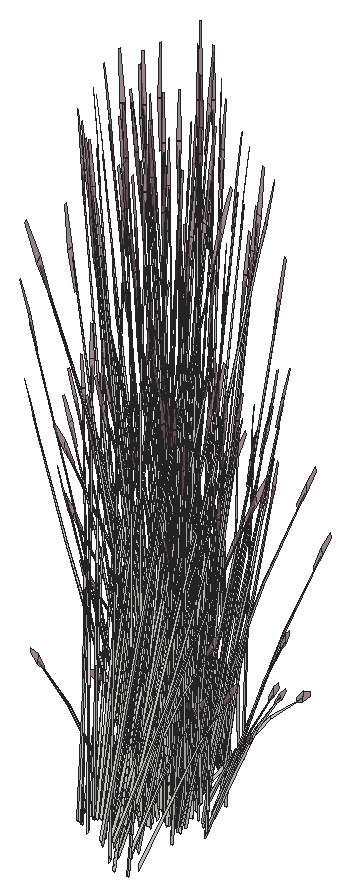
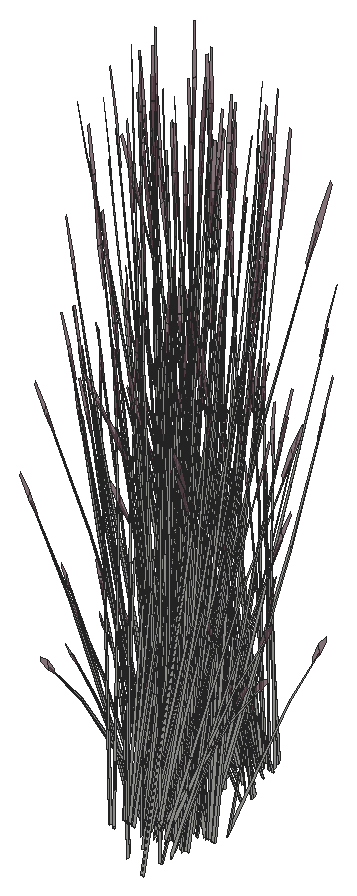
# SketchUp Ruby script. Lengths in inches.
U = 1.inch
M = Sketchup.active_model
def pt(a) = Geom::Point3d.new(a.map { |v| v * U })
def face(e, loops, mat)
  f = e.add_face(loops[0].map { |a| pt(a) })
  loops[1..].each { |l| e.add_face(l.map { |a| pt(a) }).erase! }
  f.material = f.back_material = mat if mat
  f
end
# faces: each face lists its corners as indices into pts; further lists are holes
def faces(e, pts, list, mat = nil) = list.each { |f| face(e, (f[0].is_a?(Array) ? f : [f]).map { |l| l.map { |i| pts[i] } }, mat) }
# xy, xz, yz: faces in a plane at the given z, y or x. An outline is a flat list of corners, or four numbers for a rectangle; further outlines are holes
def ring(l) = l.size == 4 ? [[l[0], l[1]], [l[2], l[1]], [l[2], l[3]], [l[0], l[3]]] : l.each_slice(2).to_a
def flat(e, list, mat, &to3) = list.each { |f| face(e, (f[0].is_a?(Array) ? f : [f]).map { |l| ring(l).map { |u, v| to3.(u, v) } }, mat) }
def xy(e, z, list, mat = nil) = flat(e, list, mat) { |x, y| [x, y, z] }
def xz(e, y, list, mat = nil) = flat(e, list, mat) { |x, z| [x, y, z] }
def yz(e, x, list, mat = nil) = flat(e, list, mat) { |y, z| [x, y, z] }
def lines(e, pts, list) = list.each { |a, b| e.add_line(pt(pts[a]), pt(pts[b])) }
# prism: a flat outline (further loops are holes) pulled along v
def prism(e, loops, v, mat = nil)
  f = face(e, loops, mat); d = Geom::Vector3d.new(v.map { |x| x * U })
  f.pushpull(f.normal.samedirection?(d) ? d.length : -d.length)
end
def box(e, o, s, mat = nil) = prism(e, [[o, [o[0] + s[0], o[1], o[2]], [o[0] + s[0], o[1] + s[1], o[2]], [o[0], o[1] + s[1], o[2]]]], [0, 0, s[2]], mat)
def at(x, y, z, deg = 0) = Geom::Transformation.translation(pt([x, y, z])) * Geom::Transformation.rotation(ORIGIN, Z_AXIS, deg.degrees)
def axes(o, x, y, z) = Geom::Transformation.new([*x, 0, *y, 0, *z, 0, *pt(o).to_a, 1])
def part(name) = M.definitions.add(name)
# library, detail: a bought-in or finely detailed component or shape, given as its bounding box
def library(name, o, s) = part(name).tap { |d| box(d.entities, o, s) }
def detail(e, o, s) = box(e.add_group.entities, o, s)
def put(e, d, t, mat = nil) = e.add_instance(d, t).tap { |i| i.material = mat if mat }
def group(e, t, mat = nil) = e.add_group.tap { |g| g.transformation = t; g.material = mat if mat }.entities
root = M.entities
M.materials.add("LightPink_Translucent").color = [144, 107, 117]
M.materials["LightPink_Translucent"].alpha = 0.75
c1 = part("blade")
p = [[2.15,0.21,22],[0,0.17,0],[0.09,0.45,0],[2.18,0.31,22],[2.29,0.31,22],[0.38,0.45,0],
  [2.48,0.24,33],[2.49,0.24,33],[2.48,0.22,33]]
faces(c1.entities,p,[[0,1,2,3],[4,5,2,3],[6,3,4,7],[8,0,3,6]])
c2 = part("seeds")
p = [[0.3,-0.1,1.38],[-0.01,-0.03,1.59],[-0.01,-0.03,0.03],[0.14,-0.07,-0.07],[0.29,-0.03,3],[0.15,0.01,3.11]]
faces(c2.entities,p,[[0,1,2,3],[1,0,4,5]],"LightPink_Translucent")
c3 = part("blade with seeds")
put(c3.entities,c1,at(0,0,0))
put(c3.entities,c2,axes([2.4,0.25,30.99],[1.5799,-0.05474,1.17369],[-0.12525,1.92788,0.29478],[-0.07173,-0.02425,1.56792]))
put(root,c3,axes([413.54,297.29,-10.12],[0,0.54355,-0.46235],[-0.57217,0,0],[0,0.1238,1.46668]))
put(root,c3,axes([412.11,297.35,-8.39],[-0.18996,-0.09365,1.59586],[0.39312,-0.39287,0.12904],[0.24502,0.17723,0.68222]))
put(root,c3,axes([412.15,296.12,-7.83],[-0.44191,-0.28242,1.28769],[0.46662,-0.43971,0.5556],[0.14258,0.26499,1.24467]))
put(root,c3,axes([408.96,297.3125,-7.3125],[0.47307,0.29971,-0.11324],[-0.27254,0.43404,-0.62851],[-0.13365,0.15087,0.95501]))
put(root,c3,axes([412.8125,298.42,-9.42],[-0.28795,-0.15629,1.06958],[0.37181,-0.1588,0.78586],[0.10029,0.13452,0.23558]))
put(root,c3,axes([411.8,298.87,-7.3125],[0.30474,-0.46525,-0.11324],[0.44133,0.26804,-0.62851],[0.15341,0.13145,0.95501]))
put(root,c3,axes([409.82,303.12,-7.6],[0.23243,-0.34529,0.05988],[0.331,0.20103,0.47138],[-0.10701,-0.1107,0.71878]))
put(root,c3,axes([408.92,303.07,-10.61],[-0.04954,0.0716,1.6421],[-0.50062,0.15438,-0.25086],[-0.12094,-0.14044,0.2797]))
put(root,c3,axes([409.75,305.04,-10.05],[-0.21003,-0.55738,-0.65031],[0.60499,-0.20074,-0.17068],[-0.02321,-0.18874,1.43544]))
put(root,c3,axes([409.2,297.67,-7.64],[0.13138,0.49631,-0.47583],[-0.49754,0.08682,-0.36857],[-0.14258,0.13331,0.91046]))
put(root,c3,axes([412.56,303.33,-10.61],[-0.07655,-0.04282,1.6421],[-0.19662,-0.47839,-0.25086],[0.13264,-0.12982,0.2797]))
put(root,c3,axes([409.79,298.24,-7.3],[0.34603,-0.28618,0.32977],[0.32756,0.32677,-0.42575],[-0.04984,0.16603,0.81462]))
put(root,c3,axes([412.38,298.82,-9.79],[0.31974,0.54466,0],[-0.53494,0.30375,-0.48057],[-0.12184,0.06918,1.52448]))
put(root,c3,axes([410.98,303.44,-7.3],[-0.15418,0.41799,0.32977],[-0.44981,-0.12192,-0.42575],[-0.04124,-0.16829,0.81462]))
put(root,c3,axes([411.4,299.25,-7.62],[0.00151,-0.06581,1.65179],[0.43826,-0.29033,-0.15608],[0.15223,0.10363,0.29231]))
put(root,c3,axes([412.89,299,-10.61],[0.03726,-0.07847,1.6421],[0.46909,-0.23111,-0.25086],[0.14221,0.11962,0.2797]))
put(root,c3,axes([412.11,296.66,-9.35],[-0.01397,-0.51177,1.31553],[0.63227,0.13266,0.557],[-0.14954,0.28003,1.24175]))
put(root,c3,axes([412.27,297.22,-10.05],[0.18752,0.49766,-0.6445],[-0.54017,0.17923,-0.16915],[0.02073,0.16852,1.42262]))
put(root,c3,axes([409.48,298.5,-7.6],[-0.42027,-0.02533,0.05988],[0.01152,-0.38243,0.47138],[-0.04398,0.14649,0.71878]))
put(root,c3,axes([409.58,303.52,-7.64],[-0.50465,0.12921,-0.47583],[-0.08828,-0.48932,-0.36857],[-0.13555,-0.14022,0.91046]))
put(root,c3,axes([412.125,303.62,-7.59],[0.36417,0.37086,0.447],[-0.38674,0.31985,0.36857],[0.06718,-0.174,0.92496]))
put(root,c3,axes([409.61,298.53,-7.59],[-0.36417,-0.37086,0.447],[0.38674,-0.31985,0.36857],[-0.06718,0.174,0.92496]))
put(root,c3,axes([412.16,298.64,-7.64],[0.50465,-0.12921,-0.47583],[0.08828,0.48932,-0.36857],[0.13555,0.14022,0.91046]))
put(root,c3,axes([409.93,303.08,-6.94],[-0.34131,0.52108,-0.12682],[-0.49429,-0.3002,-0.70393],[-0.17182,-0.14722,1.06961]))
put(root,c3,axes([412.26,303.65,-7.6],[0.42027,0.02533,0.05988],[-0.01152,0.38243,0.47138],[0.04398,-0.14649,0.71878]))
put(root,c3,axes([410.76,298.71,-7.3],[0.15418,-0.41799,0.32977],[0.44981,0.12192,-0.42575],[0.04124,0.16829,0.81462]))
put(root,c3,axes([411.95,303.91,-7.3],[-0.34603,0.28618,0.32977],[-0.32756,-0.32677,-0.42575],[0.04984,-0.16603,0.81462]))
put(root,c3,axes([412.56,304.68,-7.36],[0.26714,-0.42887,-0.66157],[0.46811,0.30479,0.07984],[0.1595,-0.15539,0.93586]))
put(root,c3,axes([409.67,303.43,-9.79],[-0.31974,-0.54466,0],[0.53494,-0.30375,-0.48057],[0.12184,-0.06918,1.52448]))
put(root,c3,axes([412.54,304.48,-7.64],[-0.13138,-0.49631,-0.47583],[0.49754,-0.08682,-0.36857],[0.14258,-0.13331,0.91046]))
put(root,c3,axes([412.86,299.13,-9.52],[-0.32795,-0.01705,0.97832],[0.21658,-0.36206,0.54015],[0.12956,0.12863,0.76741]))
put(root,c3,axes([410.37,302.78,-10.02],[-0.35341,0.31182,-0.03625],[-0.32382,-0.34152,-0.16435],[-0.0228,-0.09677,0.54209]))
put(root,c3,axes([411.91,299.04,-7.6],[-0.23243,0.34529,0.05988],[-0.331,-0.20103,0.47138],[0.10701,0.1107,0.71878]))
put(root,c3,axes([411.37,300.2,-6.74],[0.35341,-0.31182,-0.06041],[0.32382,0.34152,-0.27392],[0.0228,0.09677,0.90349]))
put(root,c3,axes([412.78,304.84,-7.3125],[-0.47307,-0.29971,-0.11324],[0.27254,-0.43404,-0.62851],[0.13365,-0.15087,0.95501]))
put(root,c3,axes([412.01,298.94,-7.59],[-0.50866,0.12474,0.447],[-0.08828,-0.48932,0.36857],[0.11963,0.14421,0.92496]))
put(root,c3,axes([409.5,297.59,-8.39],[0.09522,-0.18683,1.59586],[0.39947,0.38663,0.12904],[-0.18021,0.24097,0.68222]))
put(root,c3,axes([410.82,306.47,-8.9],[0.44194,0.21918,1.40854],[-0.43295,0.47219,0.557],[-0.19393,-0.27986,1.18082]))
put(root,c3,axes([411.79,298.25,-9.59],[0.00902,-0.18018,1.33163],[0.43127,-0.20126,-0.28638],[0.13313,0.21566,0.56934]))
put(root,c3,axes([409.9,303.51,-7.3],[0.07899,0.43781,0.32977],[-0.45153,0.11561,-0.42575],[-0.12128,-0.12546,0.81462]))
put(root,c3,axes([408.51,304.96,-10.12],[0,-0.54355,-0.46235],[0.57217,0,0],[0,-0.1238,1.46668]))
put(root,c3,axes([410.1,303.35,-10.12],[0.47863,-0.27177,-0.46235],[0.28609,0.48733,0],[0.10901,-0.0619,1.46668]))
put(root,c3,axes([412.94,304.29,-9.59],[-0.1827,-0.0161,1.33163],[-0.18717,-0.43188,-0.28638],[0.22444,-0.12218,0.56934]))
put(root,c3,axes([410.625,299.09,-7.6],[-0.37684,0.18473,0.05988],[-0.18445,-0.33686,0.47138],[0.03639,0.14849,0.71878]))
put(root,c3,axes([413.94,304.71,-7.62],[-0.0668,-0.00413,1.65179],[-0.27738,-0.44233,-0.15608],[0.11139,-0.14544,0.29231]))
put(root,c3,axes([409.61,298.64,-7.78],[-0.34603,0.28618,-0.32977],[-0.32756,-0.32677,0.42575],[-0.04984,0.16603,0.81462]))
put(root,c3,axes([408.42,298.56,-7.61],[-0.01271,0.10756,1.62908],[0.36076,0.37419,-0.25764],[-0.09444,0.17695,0.13065]))
put(root,c3,axes([409.57,298.32,-6.97],[0.56206,0.02693,-0.12569],[-0.01536,0.50991,-0.69765],[-0.03904,0.19638,1.06006]))
put(root,c3,axes([410.61,298.89,-7.3125],[0.50045,-0.25306,-0.11324],[0.24593,0.44915,-0.62851],[0.06603,0.18927,0.95501]))
put(root,c3,axes([410.76,299.05,-7.28],[-0.50393,-0.1421,0.49617],[0.17232,-0.46717,0.40911],[0.03028,0.18372,1.0267]))
put(root,c3,axes([410.67,304.47,-10.08],[0.34446,-0.40855,-0.58063],[0.42791,0.37046,-0.15239],[0.13803,-0.10191,1.28164]))
put(root,c3,axes([409.83,299.76,-9.42],[-0.01324,-0.32319,1.06958],[0.33072,0.23052,0.78586],[-0.06504,0.15405,0.23558]))
put(root,c3,axes([413.15,303.5,-9.42],[-0.17034,0.27669,1.06958],[-0.14642,-0.37174,0.78586],[0.14069,-0.09315,0.23558]))
put(root,c3,axes([410.7,298.98,-10.61],[0.08277,-0.02958,1.6421],[0.49786,0.16279,-0.25086],[0.01456,0.18348,0.2797]))
put(root,c3,axes([412.91,304.54,-7.78],[0.44516,-0.07768,-0.32977],[0.11755,0.44407,0.42575],[0.12757,-0.11927,0.81462]))
put(root,c3,axes([409.96,298.51,-7.34],[0.3661,0.36521,-0.52818],[-0.38674,0.31985,-0.40911],[-0.0557,0.18556,1.01061]))
put(root,c3,axes([410.07,305.18,-9.94],[0.24813,-0.48978,-0.41661],[0.51557,0.23571,0.2005],[0,-0.1129,1.33761]))
put(root,c3,axes([410.3,304.9375,-9.52],[-0.05959,-0.62022,-0.27094],[0.62068,-0.0375,-0.46562],[0.1093,-0.08261,1.4872]))
put(root,c3,axes([409.56,299.06,-9.37],[0.46459,-0.09625,0.0606],[0.10681,0.38778,-0.80367],[-0.02945,0.1963,0.72038]))
put(root,c3,axes([411.04,298.86,-7.64],[0.50273,0.13626,-0.47583],[-0.17232,0.46717,-0.36857],[0.0461,0.18809,0.91046]))
put(root,c3,axes([408.76,304.97,-10.11],[0.35699,-0.33913,-0.28847],[0.35699,0.33913,0.28847],[0,-0.10923,1.29413]))
put(root,c3,axes([411.33,297.9,-8.39],[-0.1169,-0.17452,1.59586],[0.54019,-0.14692,0.12904],[0.12209,0.27397,0.68222]))
put(root,c3,axes([408.61,303.35,-10.02],[-0.14753,0.44383,-0.03625],[-0.45406,-0.13653,-0.16435],[-0.06894,-0.07259,0.54209]))
put(root,c3,axes([412.55,304.8,-7.3],[-0.44516,0.07768,0.32977],[-0.11755,-0.44407,-0.42575],[0.12757,-0.11927,0.81462]))
put(root,c3,axes([410.01,305.59,-9.52],[-0.57594,-0.25935,-0.27094],[0.27732,-0.5474,-0.46562],[-0.0181,-0.1344,1.4872]))
put(root,c3,axes([408.37,305.37,-9.79],[-0.63949,0,0],[0,-0.60749,-0.48057],[0,-0.13836,1.52448]))
put(root,c3,axes([410.8125,299.15,-7.78],[-0.15418,0.41799,-0.32977],[-0.44981,-0.12192,0.42575],[0.04124,0.16829,0.81462]))
put(root,c3,axes([410.21,303.57,-10.11],[0.47712,0.13449,-0.28847],[-0.12013,0.47362,0.28847],[0.09619,-0.05462,1.29413]))
put(root,c3,axes([409.84,298.34,-7.03],[-0.01331,0.50278,-0.73435],[-0.56035,-0.03377,0.08862],[-0.05914,0.213,1.03881]))
put(root,c3,axes([408.38,299.66,-7.62],[0.05802,-0.03282,1.65179],[0.47954,0.21828,-0.15608],[-0.01127,0.18175,0.29231]))
put(root,c3,axes([410.37,297.99,-8.39],[-0.01252,-0.20862,1.59586],[0.54251,0.1384,0.12904],[-0.03356,0.2973,0.68222]))
put(root,c3,axes([412.95,304.73,-7.6],[0.35109,0.22859,0.05988],[-0.2044,0.32553,0.47138],[0.11256,-0.10524,0.71878]))
put(root,c3,axes([412.85,304.63,-7.59],[0.12683,0.50025,0.447],[-0.49754,0.08682,0.36857],[0.14663,-0.11765,0.92496]))
put(root,c3,axes([414.19,305.24,-7.61],[0.07097,-0.08279,1.62908],[-0.09083,-0.50786,-0.25764],[0.17806,-0.09629,0.13065]))
put(root,c3,axes([410.86,298.77,-7.36],[0.24409,0.44196,-0.66157],[-0.50245,0.2463,0.07984],[0.05708,0.21354,0.93586]))
put(root,c3,axes([408.87,305.21,-9.83],[-0.47569,0.45698,0.2864],[-0.47598,-0.45217,-0.33981],[-0.01661,-0.12977,1.53541]))
put(root,c3,axes([409.45,299.47,-9.59],[0.16138,-0.08575,1.33163],[0.39845,0.25854,-0.28638],[-0.1186,0.22371,0.56934]))
put(root,c3,axes([410.49,299.89,-7.61],[0.06483,0.08753,1.62908],[0.52315,0.03439,-0.25764],[0.05261,0.19303,0.13065]))
put(root,c3,axes([410.38,305.42,-9.73],[0.57623,0.26344,0.22409],[-0.27732,0.5474,0.46562],[0,-0.12618,1.49497]))
put(root,c3,axes([410.15,306.16,-9.73],[0.13555,-0.64407,-0.21817],[0.64269,0.11227,0.47743],[-0.1123,-0.08895,1.45677]))
put(root,c3,axes([409,304.1,-7.3],[0.29098,0.34031,0.32977],[-0.33226,0.32215,-0.42575],[-0.16881,-0.04902,0.81462]))
put(root,c3,axes([410.19,305.06,-9.47],[-0.55535,0.03355,0.41661],[-0.05022,-0.55698,-0.2005],[0.09942,-0.05645,1.33761]))
put(root,c3,axes([408.76,305.46,-9.69],[0,0.54355,0.46235],[-0.57217,0,0],[0,-0.1238,1.46668]))
put(root,c3,axes([412.8,306.01,-7.3125],[-0.25732,-0.49218,-0.11324],[0.45669,-0.24187,-0.62851],[0.19245,-0.06494,0.95501]))
put(root,c3,axes([412.77,305.59,-7.64],[0.13855,-0.49442,-0.47583],[0.47502,0.16947,-0.36857],[0.19125,-0.04534,0.91046]))
put(root,c3,axes([409.65,299.05,-8.87],[0.01124,-0.2806,1.43727],[0.50537,0.14821,0.19862],[-0.04379,0.29905,0.67868]))
put(root,c3,axes([412.02,303.57,-9.79],[0.31974,-0.54466,0],[0.53494,0.30375,-0.48057],[0.12184,0.06918,1.52448]))
put(root,c3,axes([410.11,305.9,-9.94],[-0.30722,-0.45622,-0.41661],[0.46535,-0.32126,0.2005],[-0.09942,-0.05645,1.33761]))
put(root,c3,axes([410.17,305.26,-9.8],[0.22235,0.6078,0.42607],[-0.63531,0.21135,0.16719],[0.00776,-0.11168,1.47927]))
put(root,c3,axes([413.28,305.72,-10.15],[-0.32938,0.06523,1.31842],[-0.05243,-0.51922,0.07547],[0.2307,-0.07859,0.75023]))
put(root,c3,axes([413.88,305.26,-9.89],[-0.31706,-0.34757,-0.06041],[0.34725,-0.31847,-0.27392],[0.09839,-0.02242,0.90349]))
put(root,c3,axes([410.0625,305.74,-9.47],[-0.24813,0.48978,0.41661],[-0.51557,-0.23571,-0.2005],[0,-0.1129,1.33761]))
put(root,c3,axes([410.97,305.31,-9.95],[0,-0.62892,0],[0.63949,0,0],[0,0,1.6711]))
put(root,c3,axes([411.75,303.86,-9.69],[-0.47863,-0.27177,0.46235],[0.28609,-0.48733,0],[0.10901,0.0619,1.46668]))
put(root,c3,axes([412.68,305.77,-7.36],[0.44939,-0.24006,-0.66157],[0.25044,0.49415,0.07984],[0.21713,-0.05613,0.93586]))
put(root,c3,axes([410.67,304.91,-9.8],[-0.42403,0.49328,0.42607],[-0.50377,-0.43543,0.16719],[0.10223,-0.04923,1.47927]))
put(root,c3,axes([411.13,305.8,-9.86],[-0.47569,-0.46784,-0.05709],[0.47598,-0.46812,0],[-0.01661,-0.01634,1.63492]))
put(root,c3,axes([409.93,304.1,-9.7],[-0.14774,0.54019,0.16428],[-0.54062,-0.15287,0.32672],[0.09339,-0.00263,1.49371]))
put(root,c3,axes([412.62,305.86,-7.3],[-0.42502,-0.15163,0.32977],[0.12396,-0.44238,-0.42575],[0.17112,-0.04056,0.81462]))
put(root,c3,axes([408.99,309.54,-8.39],[0.1169,0.17452,1.59586],[-0.54019,0.14692,0.12904],[-0.12209,-0.27397,0.68222]))
put(root,c3,axes([409.71,304.54,-10.52],[-0.50338,0.21762,1.20058],[-0.16022,-0.62439,0.4665],[0.30911,0.01039,1.36553]))
put(root,c3,axes([411.0625,304.7,-9.5625],[0.09866,-0.48509,0.13483],[0.48202,0.0842,-0.38503],[0.08772,0.04981,1.18024]))
put(root,c3,axes([409.88,308.38,-7.61],[-0.07822,-0.07621,1.62908],[-0.52201,0.04832,-0.25764],[-0.08331,-0.18228,0.13065]))
put(root,c3,axes([410.23,305.85,-9.8],[0.64638,0.11452,0.42607],[-0.13155,0.64678,0.16719],[-0.09446,-0.06245,1.47927]))
put(root,c3,axes([413.64,305.39,-10.61],[-0.02673,-0.08252,1.6421],[0.18538,-0.48271,-0.25086],[0.187,-0.00694,0.2797]))
put(root,c3,axes([411.09,309.28,-9.59],[-0.14537,0.11002,1.33163],[-0.43536,-0.19256,-0.28638],[0.0807,-0.23948,0.56934]))
put(root,c3,axes([410.43,309.67,-7.36],[-0.24409,-0.44196,-0.66157],[0.50245,-0.2463,0.07984],[-0.05708,-0.21354,0.93586]))
put(root,c3,axes([410.86,304.83,-9.47],[-0.30722,-0.45622,0.41661],[0.46535,-0.32126,-0.2005],[0.09942,0.05645,1.33761]))
put(root,c3,axes([408.84,309.07,-9.59],[-0.03097,0.17781,1.33163],[-0.45273,0.14885,-0.28638],[-0.10583,-0.22982,0.56934]))
put(root,c3,axes([409.27,306.92,-10.11],[-0.12013,-0.47362,-0.28847],[0.47712,-0.13449,0.28847],[-0.09619,-0.05462,1.29413]))
put(root,c3,axes([410.01,308.69,-10.61],[-0.08578,0.01958,1.6421],[-0.47437,-0.22044,-0.25086],[0.00796,-0.18387,0.2797]))
put(root,c3,axes([409.88,306.89,-9.7],[0.54955,-0.14427,0.16428],[0.1357,0.53689,0.32672],[-0.04901,-0.07823,1.49371]))
put(root,c3,axes([411.01,304.86,-9.52],[0.51635,-0.36087,-0.27094],[0.34336,0.5099,-0.46562],[0.1274,0.05178,1.4872]))
put(root,c3,axes([413.07,305.8125,-7.78],[0.42502,0.15163,-0.32977],[-0.12396,0.44238,0.42575],[0.17112,-0.04056,0.81462]))
put(root,c3,axes([409.13,307.12,-10.12],[-0.47863,-0.27177,-0.46235],[0.28609,-0.48733,0],[-0.10901,-0.0619,1.46668]))
put(root,c3,axes([412.3125,303.9,-10.12],[0.47863,0.27177,-0.46235],[-0.28609,0.48733,0],[0.10901,0.0619,1.46668]))
put(root,c3,axes([411.44,310.1,-7.36],[0.01331,-0.50278,-0.66157],[0.56035,0.03377,0.07984],[0.05914,-0.213,0.93586]))
put(root,c3,axes([411.41,305.45,-9.95],[0.57217,0,0],[0,0.56272,0],[0,0,1.66132]))
put(root,c3,axes([410.4375,306.16,-9.52],[-0.51635,0.36087,-0.27094],[-0.34336,-0.5099,-0.46562],[-0.1274,-0.05178,1.4872]))
put(root,c3,axes([411.57,304.13,-9.7],[-0.54955,0.14427,0.16428],[-0.1357,-0.53689,0.32672],[0.04901,0.07823,1.49371]))
put(root,c3,axes([412.23,309.3125,-7.61],[-0.00494,-0.10818,1.62908],[-0.41695,-0.31265,-0.25764],[0.06446,-0.18952,0.13065]))
put(root,c3,axes([410.47,309.29,-7.78],[0.15418,-0.41799,-0.32977],[0.44981,0.12192,0.42575],[-0.04124,-0.16829,0.81462]))
put(root,c3,axes([410.8125,309.84,-8.39],[-0.09522,0.18683,1.59586],[-0.39947,-0.38663,0.12904],[0.18021,-0.24097,0.68222]))
put(root,c3,axes([412.11,308.92,-7.62],[-0.05194,0.04152,1.65179],[-0.50886,-0.14007,-0.15608],[-0.01842,-0.18118,0.29231]))
put(root,c3,axes([411.91,305.26,-8.39],[-0.21212,0.01231,1.59586],[0.14072,-0.53355,0.12904],[0.3023,0.033,0.68222]))
put(root,c3,axes([412.18,304.1,-10.11],[0.12013,0.47362,-0.28847],[-0.47712,0.13449,0.28847],[0.09619,0.05462,1.29413]))
put(root,c3,axes([410.24,309.58,-7.64],[-0.50273,-0.13626,-0.47583],[0.17232,-0.46717,-0.36857],[-0.0461,-0.18809,0.91046]))
put(root,c3,axes([410.56,308.41,-9.42],[0.06561,0.31695,1.06958],[-0.36394,-0.17555,0.78586],[0.03916,-0.16229,0.23558]))
put(root,c3,axes([413,306,-7.6],[0.18783,0.37061,0.05988],[-0.34252,0.1814,0.47138],[0.15099,-0.03579,0.71878]))
put(root,c3,axes([411.33,309.93,-7.64],[-0.3661,-0.36521,-0.47583],[0.38674,-0.31985,-0.36857],[0.0557,-0.18556,0.91046]))
put(root,c3,axes([411.22,305.16,-9.78],[-0.64638,-0.11452,0.45814],[0.13155,-0.64678,0.17978],[0.09446,0.06245,1.59061]))
put(root,c3,axes([412.97,305.87,-7.59],[-0.14449,0.4956,0.447],[-0.47502,-0.16947,0.36857],[0.1868,-0.02978,0.92496]))
put(root,c3,axes([410.71,306.76,-9.95],[-0.16686,-0.46861,0],[0.47648,-0.16411,0],[0,0,1.4375]))
put(root,c3,axes([409.34,308.13,-7.62],[-0.00954,0.06515,1.65179],[-0.47055,0.23645,-0.15608],[-0.13847,-0.12087,0.29231]))
put(root,c3,axes([410.39,306.32,-9.5625],[-0.09866,0.48509,0.13483],[-0.48202,-0.0842,-0.38503],[-0.08772,-0.04981,1.18024]))
put(root,c3,axes([411.33,306.7,-9.97],[0.53691,-0.18442,-0.17877],[0.18866,0.53125,0.00007],[0.05927,-0.02038,1.61933]))
put(root,c3,axes([411.52,306.92,-9.7],[0.14774,-0.54019,0.16428],[0.54062,0.15287,0.32672],[-0.09339,0.00263,1.49371]))
put(root,c3,axes([411.39,305.69,-9.9375],[0.35699,0.35109,0],[-0.35699,0.35109,0],[0,0,1.57621]))
put(root,c3,axes([409.24,309.29,-7.26],[0.56969,-0.13971,0.50064],[0.09887,0.54803,0.4128],[-0.13398,-0.16152,1.03595]))
put(root,c3,axes([412.36,305.54,-9.7],[-0.40181,-0.39593,0.16428],[0.40492,-0.38402,0.32672],[-0.04438,0.08086,1.49371]))
put(root,c3,axes([410.53,309.39,-7.59],[0.50393,0.1421,0.447],[-0.17232,0.46717,0.36857],[-0.03028,-0.18372,0.92496]))
put(root,c3,axes([411.62,304.94,-10.08],[0.53199,0.08911,-0.58063],[-0.11226,0.54969,-0.15239],[0.15876,0.06661,1.28164]))
put(root,c3,axes([410.67,309.55,-7.3125],[-0.50045,0.25306,-0.11324],[-0.24593,-0.44915,-0.62851],[-0.06603,-0.18927,0.95501]))
put(root,c3,axes([413.97,305.9,-9.42],[-0.31598,0.08973,1.06958],[0.14873,-0.37085,0.78586],[0.16763,0.02538,0.23558]))
put(root,c3,axes([411.71,310.125,-7.3125],[-0.56206,-0.02693,-0.11324],[0.01536,-0.50991,-0.62851],[0.03904,-0.19638,0.95501]))
put(root,c3,axes([411.67,309.8,-7.78],[0.34603,-0.28618,-0.32977],[0.32756,0.32677,0.42575],[0.04984,-0.16603,0.81462]))
put(root,c3,axes([408.68,308.79,-9.42],[0.26677,0.18918,1.06958],[-0.38851,0.11372,0.78586],[-0.08313,-0.14539,0.23558]))
put(root,c3,axes([410.66,309.35,-7.6],[0.37684,-0.18473,0.05988],[0.18445,0.33686,0.47138],[-0.03639,-0.14849,0.71878]))
put(root,c3,axes([409.18,309.44,-7.78],[-0.07899,-0.43781,-0.32977],[0.45153,-0.11561,0.42575],[-0.12128,-0.12546,0.81462]))
put(root,c3,axes([410.59,306.97,-9.95],[-0.51557,-0.24403,0],[0.24813,-0.50705,0],[0,0,1.51513]))
put(root,c3,axes([411.02,306.32,-9.7],[-0.49938,-0.43748,-0.23459],[0.42021,-0.49126,0.51337],[-0.13447,0.05118,1.56642]))
put(root,c3,axes([409.7,307.16,-9.69],[0.47863,0.27177,0.46235],[-0.28609,0.48733,0],[-0.10901,-0.0619,1.46668]))
put(root,c3,axes([411.39,305.28,-9.47],[0.24813,-0.48978,0.41661],[0.51557,0.23571,-0.2005],[0,0.1129,1.33761]))
put(root,c3,axes([413.82,307.47,-7.62],[-0.04624,-0.04758,1.65179],[0.10116,-0.51007,-0.15608],[0.18215,-0.03259,0.29231]))
put(root,c3,axes([411.29,305.5625,-9.87],[0,0.62861,-0.05249],[-0.63949,0,0],[0,0.01975,1.67027]))
put(root,c3,axes([411.34,305.12,-9.94],[0.30722,0.45622,-0.41661],[-0.46535,0.32126,0.2005],[0.09942,0.05645,1.33761]))
put(root,c3,axes([413.42,307.04,-8.34],[-0.09788,-0.45691,-0.03251],[0.46264,-0.10504,-0.14742],[0.09661,0.02897,0.48626]))
put(root,c3,axes([409.43,307.45,-9.79],[-0.31974,0.54466,0],[-0.53494,-0.30375,-0.48057],[-0.12184,-0.06918,1.52448]))
put(root,c3,axes([412.22,307.03,-7.3125],[0.02738,-0.55277,-0.11324],[0.51847,0.01511,-0.62851],[0.19968,0.0384,0.95501]))
put(root,c3,axes([409.37,309.4,-7.6],[0.23243,-0.34529,0.05988],[0.331,0.20103,0.47138],[-0.10701,-0.1107,0.71878]))
put(root,c3,axes([412.69,305.55,-9.69],[0,-0.54355,0.46235],[0.57217,0,0],[0,0.1238,1.46668]))
put(root,c3,axes([411.26,305.96,-9.47],[0.55535,-0.03355,0.41661],[0.05022,0.55698,-0.2005],[-0.09942,0.05645,1.33761]))
put(root,c3,axes([411.6,305.39,-9.5625],[0.47648,-0.15851,0.13483],[0.16686,0.45265,-0.38503],[0,0.09962,1.18024]))
put(root,c3,axes([409.3,311.33,-10.05],[-0.21003,-0.55738,-0.65031],[0.60499,-0.20074,-0.17068],[-0.02321,-0.18874,1.43544]))
put(root,c3,axes([412.11,309.62,-10.61],[-0.07655,-0.04282,1.6421],[-0.19662,-0.47839,-0.25086],[0.13264,-0.12982,0.2797]))
put(root,c3,axes([412.14,306.8125,-7.3],[-0.29098,-0.34031,0.32977],[0.33226,-0.32215,-0.42575],[0.16881,0.04902,0.81462]))
put(root,c3,axes([410.76,306.23,-9.94],[-0.55535,0.03355,-0.41661],[-0.05022,-0.55698,0.2005],[-0.09942,0.05645,1.33761]))
put(root,c3,axes([410.52,309.73,-7.3],[-0.15418,0.41799,0.32977],[-0.44981,-0.12192,-0.42575],[-0.04124,-0.16829,0.81462]))
put(root,c3,axes([413.375,306.5,-9.59],[-0.12317,-0.13368,1.33163],[0.16025,-0.44223,-0.28638],[0.24919,0.05991,0.56934]))
put(root,c3,axes([411.67,309.91,-7.59],[0.36417,0.37086,0.447],[-0.38674,0.31985,0.36857],[0.06718,-0.174,0.92496]))
put(root,c3,axes([411.81,309.94,-7.6],[0.42027,0.02533,0.05988],[-0.01152,0.38243,0.47138],[0.04398,-0.14649,0.71878]))
put(root,c3,axes([411.17,306.98,-9.95],[0.51557,0.24403,0],[-0.24813,0.50705,0],[0,0,1.62917]))
put(root,c3,axes([411.49,310.2,-7.3],[-0.34603,0.28618,0.32977],[-0.32756,-0.32677,-0.42575],[0.04984,-0.16603,0.81462]))
put(root,c3,axes([412.1,310.97,-7.36],[0.26714,-0.42887,-0.66157],[0.46811,0.30479,0.07984],[0.1595,-0.15539,0.93586]))
put(root,c3,axes([412.67,306.7,-7.61],[0.10971,-0.00919,1.62908],[0.30091,-0.42228,-0.25764],[0.19514,0.05574,0.13065]))
put(root,c3,axes([411.38,307.52,-9.96],[-0.31576,-0.54657,-0.04789],[0.53494,-0.30375,0.48057],[-0.13182,0.05204,1.52373]))
put(root,c3,axes([409.22,309.72,-9.79],[-0.31974,-0.54466,0],[0.53494,-0.30375,-0.48057],[0.12184,-0.06918,1.52448]))
put(root,c3,axes([412.09,310.77,-7.64],[-0.13138,-0.49631,-0.47583],[0.49754,-0.08682,-0.36857],[0.14258,-0.13331,0.91046]))
put(root,c3,axes([411.27,306.2,-9.5625],[0.37783,0.32657,0.13483],[-0.31516,0.36844,-0.38503],[-0.08772,0.04981,1.18024]))
